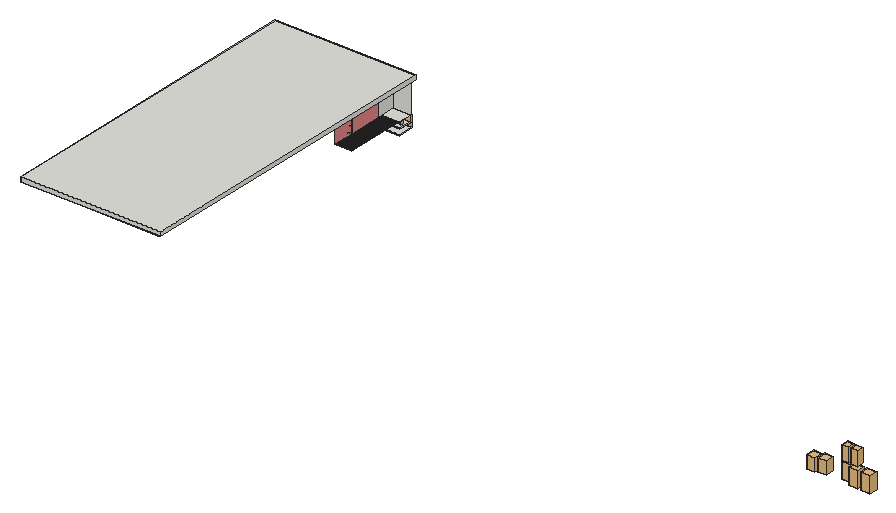
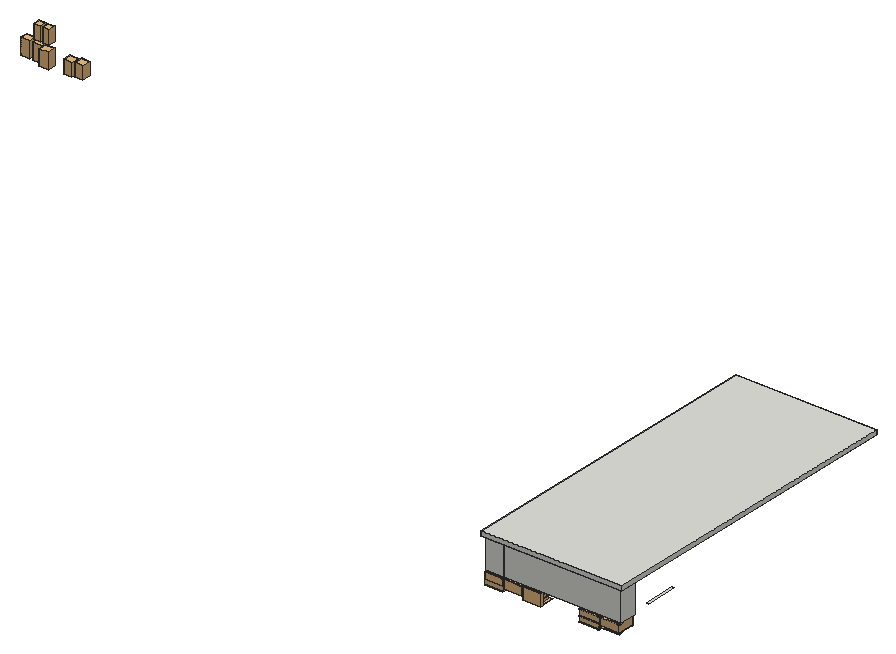
# SketchUp Ruby script. Lengths in inches.
U = 1.inch
M = Sketchup.active_model
def pt(a) = Geom::Point3d.new(a.map { |v| v * U })
def face(e, loops, mat)
  f = e.add_face(loops[0].map { |a| pt(a) })
  loops[1..].each { |l| e.add_face(l.map { |a| pt(a) }).erase! }
  f.material = f.back_material = mat if mat
  f
end
# faces: each face lists its corners as indices into pts; further lists are holes
def faces(e, pts, list, mat = nil) = list.each { |f| face(e, (f[0].is_a?(Array) ? f : [f]).map { |l| l.map { |i| pts[i] } }, mat) }
# xy, xz, yz: faces in a plane at the given z, y or x. An outline is a flat list of corners, or four numbers for a rectangle; further outlines are holes
def ring(l) = l.size == 4 ? [[l[0], l[1]], [l[2], l[1]], [l[2], l[3]], [l[0], l[3]]] : l.each_slice(2).to_a
def flat(e, list, mat, &to3) = list.each { |f| face(e, (f[0].is_a?(Array) ? f : [f]).map { |l| ring(l).map { |u, v| to3.(u, v) } }, mat) }
def xy(e, z, list, mat = nil) = flat(e, list, mat) { |x, y| [x, y, z] }
def xz(e, y, list, mat = nil) = flat(e, list, mat) { |x, z| [x, y, z] }
def yz(e, x, list, mat = nil) = flat(e, list, mat) { |y, z| [x, y, z] }
def lines(e, pts, list) = list.each { |a, b| e.add_line(pt(pts[a]), pt(pts[b])) }
# prism: a flat outline (further loops are holes) pulled along v
def prism(e, loops, v, mat = nil)
  f = face(e, loops, mat); d = Geom::Vector3d.new(v.map { |x| x * U })
  f.pushpull(f.normal.samedirection?(d) ? d.length : -d.length)
end
def box(e, o, s, mat = nil) = prism(e, [[o, [o[0] + s[0], o[1], o[2]], [o[0] + s[0], o[1] + s[1], o[2]], [o[0], o[1] + s[1], o[2]]]], [0, 0, s[2]], mat)
def at(x, y, z, deg = 0) = Geom::Transformation.translation(pt([x, y, z])) * Geom::Transformation.rotation(ORIGIN, Z_AXIS, deg.degrees)
def axes(o, x, y, z) = Geom::Transformation.new([*x, 0, *y, 0, *z, 0, *pt(o).to_a, 1])
def part(name) = M.definitions.add(name)
# library, detail: a bought-in or finely detailed component or shape, given as its bounding box
def library(name, o, s) = part(name).tap { |d| box(d.entities, o, s) }
def detail(e, o, s) = box(e.add_group.entities, o, s)
def put(e, d, t, mat = nil) = e.add_instance(d, t).tap { |i| i.material = mat if mat }
def group(e, t, mat = nil) = e.add_group.tap { |g| g.transformation = t; g.material = mat if mat }.entities
root = M.entities
M.materials.add("Generic\#1").color = [224, 133, 133]
M.materials.add("[0036_BurlyWood]").color = [222, 184, 135]
M.materials.add("[0134_DimGray]").color = [105, 105, 105]
M.materials.add("[0136_Charcoal]").color = [35, 35, 35]
M.materials.add("[Color M00]").color = [255, 255, 255]
c1 = library("Group\#42",[-0.5,-0.5,-0.1],[27.07,5.46,0.2])
c2 = library("Group\#45",[-0.5,-0.5,0],[25.0625,2.8125,15.73])
c3 = library("KITCHEN+ITEMS+(22)",[-8.24,-11.1,-0.01],[16.86,31.33,9.97])
c4 = library("Food+jars (2)",[-11.5,-3.52,0],[30.82,7.02,10])
c5 = library("Group\#41",[-0.5,-0.5,-0.1],[27.07,6.0625,0.2])
c6 = library("Group\#46",[-0.5,-0.5,0],[25.0625,7.1875,12.03])
c7 = library("KITCHEN+ITEMS+(3)",[-2.27,-9.02,0],[4.03,10.9,5.45])
c8 = library("Stocked cup rack",[0,0,0],[12.28,12.62,7.74])
c9 = library("Group\#47",[-0.5,-0.5,0],[25.0625,2.47,8.52])
c10 = library("Group\#43",[-0.5,-0.5,-0.1],[27.07,5.46,0.2])
c11 = library("Group\#8",[-92.73,64.66,378.72],[126.77,111.9,197.69])
c12 = library("Group\#3",[-457.8,68.7,378.69],[103.44,103.46,159.72])
c13 = library("Group\#12",[309.63,77.04,613.73],[136.79,86.78,171.39])
c14 = library("filizanka,+spodek+zestaw",[-38.08,-53.17,0],[37.3,56.83,6.3])
c15 = library("Food+jars (1)",[-3.15,-4.1,0],[15.4,16.05,11.47])
c16 = library("Group\#40",[-0.5,-0.5,-0.1],[27.07,5.5625,0.2])
c17 = library("Group\#44",[-0.5,-0.5,-0.1],[27.07,3.75,0.2])
c18 = part("Group\#105")
prism(c18.entities,[[[0.55,0,1.11],[0.51,0,1.03],[0.44,0,0.97],[0.36,0,0.9375],[0.28,0,0.92],[0.19,0,0.9375],[0.11,0,0.97],[0.05,0,1.03],[0,0,1.11],[0,0,0],[0.55,0,0]]],[0,0.79,0])
c19 = part("Cabinet bar pull")
put(c19.entities,c18,axes([0,1.42,1.36],[0,0,-1],[1,0,0],[0,-1,0]))
g1 = group(c19.entities,at(0,1.42,1.36))
prism(g1,[[[0,-1.28,-0.57],[0,-1.32,-0.53],[0,-1.35,-0.49],[0,-1.38,-0.4375],[0,-1.4,-0.39],[0,-1.41,-0.33],[0,-1.42,-0.28],[0,-1.41,-0.22],[0,-1.4,-0.17],[0,-1.38,-0.11],[0,-1.35,-0.0625],[0,-1.32,-0.02],[0,-1.28,0.02],[0,-1.19,0.02],[0,-1.11,0],[0,-1.03,-0.05],[0,-0.97,-0.11],[0,-0.9375,-0.19],[0,-0.92,-0.28],[0,-0.9375,-0.36],[0,-0.97,-0.44],[0,-1.03,-0.51],[0,-1.11,-0.55],[0,-1.19,-0.57]]],[13.07,0,0])
put(c19.entities,c18,axes([12.28,1.42,1.36],[0,0,-1],[1,0,0],[0,-1,0]))
c20 = library("10 (1)",[26.65,-5.45,122.92],[1.37,1.38,0.36])
c21 = library("Group\#4",[-210.76,89.58,378.69],[103.46,103.45,159.72])
c22 = library("Group\#2",[-332.7,68.71,378.69],[103.45,103.45,159.72])
c23 = library("Group\#9",[51.24,128.79,378.72],[113.79,95.47,197.69])
c24 = library("Group\#10",[179.9,72.7,378.72],[113.8,95.46,197.69])
c25 = library("Group\#11",[327.72,72.7,378.72],[113.79,95.46,197.69])
c26 = library("Group\#19",[85.42,84.74,613.85],[84,84,172.42])
c27 = library("Group\#20",[193.57,84.74,613.85],[84,84,172.39])
xy(root,63.79,[[166.14,409.25,190.2,429.57]],"[0036_BurlyWood]")
xy(root,64.03,[[36.39,410.57,62.46,425.11]])
xy(root,64.04,[[114.85,409.25,138.91,427.75]])
xy(root,64.85,[[166.14,409.25,190.2,429.57],[36.39,410.57,62.46,429.57]])
xy(root,64.85,[[114.85,409.25,138.91,429.57]],"[0036_BurlyWood]")
xy(root,67.74,[[140.5,407.75,164.56,423.38]],"[0036_BurlyWood]")
xy(root,67.8,[[8.77,407.75,34.84,424.5]],"[0036_BurlyWood]")
xy(root,68.58,[[140.5,407.75,164.56,429.57]])
xy(root,69.36,[[8.77,407.75,34.84,429.57]],"[0036_BurlyWood]")
xy(root,71.25,[[166.14,409.25,190.2,428.1]],"[0036_BurlyWood]")
xy(root,71.5,[[114.85,409.25,138.91,427.75],[36.39,410.57,62.46,425.11]])
xy(root,72.3125,[[166.14,409.25,190.2,429.57]])
xy(root,72.3125,[[114.85,409.25,138.91,429.57]],"[0036_BurlyWood]")
xy(root,72.32,[[36.39,410.57,62.46,429.57]])
xy(root,79.77,[[114.85,407.75,138.91,427.75],[140.5,407.75,164.56,423.38],[166.14,407.75,166.97,429.57],[166.97,407.75,190.2,428.1]],"[0036_BurlyWood]")
xy(root,79.79,[[8.77,407.75,34.84,425],[36.39,407.75,62.46,426.82]],"[0036_BurlyWood]")
xy(root,80.5625,[[7.99,407.75,166.97,427.75],[166.97,407.75,191,427.75]])
xy(root,80.5625,[[166.97,328.41,166.97,357.08,167.27,357.08,167.27,357.38,166.97,357.38,166.97,407.75,191,407.75,191,328.41],[7.99,403.75,7.99,407.75,166.97,407.75,166.97,403.75,135.48,403.75,135.48,404.05,135.18,404.05,135.18,403.75,103.68,403.75,103.68,404.05,103.38,404.05,103.38,403.75,71.88,403.75,71.88,404.05,71.58,404.05,71.58,403.75,40.09,403.75,40.09,404.05,39.79,404.05,39.79,403.75]],"[0136_Charcoal]")
xy(root,86.5625,[[4.74,342.29,7.99,384.54]])
xy(root,122.5625,[[4.74,0,4.74,431,194.24,431,194.24,0,191,0,191,427.75,7.99,427.75,7.99,0],[166.97,311,166.97,357.08,167.27,357.08,167.27,357.38,166.97,357.38,166.97,427.75,191,427.75,191,311],[7.99,403.75,7.99,427.75,166.97,427.75,166.97,403.75,135.48,403.75,135.48,404.05,135.18,404.05,135.18,403.75,103.68,403.75,103.68,404.05,103.38,404.05,103.38,403.75,71.88,403.75,71.88,404.05,71.58,404.05,71.58,403.75,40.09,403.75,40.09,404.05,39.79,404.05,39.79,403.75]])
xy(root,122.5625,[[[7.99,0,7.99,403.75,39.79,403.75,39.79,404.05,40.09,404.05,40.09,403.75,71.58,403.75,71.58,404.05,71.88,404.05,71.88,403.75,103.38,403.75,103.38,404.05,103.68,404.05,103.68,403.75,135.18,403.75,135.18,404.05,135.48,404.05,135.48,403.75,166.97,403.75,166.97,357.38,167.27,357.38,167.27,357.08,166.97,357.08,166.97,311,191,311,191,0],[33.53,377.24,34.16,377.32,34.75,377.57,35.25,377.95,35.64,378.46,35.88,379.05,35.97,379.68,35.88,380.31,35.64,380.9,35.25,381.4,34.75,381.79,34.16,382.03,33.53,382.11,32.9,382.03,32.31,381.79,31.81,381.4,31.42,380.9,31.17,380.31,31.09,379.68,31.17,379.05,31.42,378.46,31.81,377.95,32.31,377.57,32.9,377.32],[89.72,377.24,90.35,377.32,90.94,377.57,91.44,377.95,91.83,378.46,92.07,379.05,92.15,379.68,92.07,380.31,91.83,380.9,91.44,381.4,90.94,381.79,90.35,382.03,89.72,382.11,89.09,382.03,88.5,381.79,87.99,381.4,87.61,380.9,87.36,380.31,87.28,379.68,87.36,379.05,87.61,378.46,87.99,377.95,88.5,377.57,89.09,377.32],[141.03,377.24,141.66,377.32,142.25,377.57,142.75,377.95,143.14,378.46,143.38,379.05,143.47,379.68,143.38,380.31,143.14,380.9,142.75,381.4,142.25,381.79,141.66,382.03,141.03,382.11,140.4,382.03,139.81,381.79,139.31,381.4,138.92,380.9,138.67,380.31,138.59,379.68,138.67,379.05,138.92,378.46,139.31,377.95,139.81,377.57,140.4,377.32]]],"[Color M00]")
xy(root,123.25,[[33.53,377.24,32.9,377.32,32.31,377.57,31.81,377.95,31.42,378.46,31.17,379.05,31.09,379.68,31.17,380.31,31.42,380.9,31.81,381.4,32.31,381.79,32.9,382.03,33.53,382.11,34.16,382.03,34.75,381.79,35.25,381.4,35.64,380.9,35.88,380.31,35.97,379.68,35.88,379.05,35.64,378.46,35.25,377.95,34.75,377.57,34.16,377.32],[89.72,377.24,89.09,377.32,88.5,377.57,87.99,377.95,87.61,378.46,87.36,379.05,87.28,379.68,87.36,380.31,87.61,380.9,87.99,381.4,88.5,381.79,89.09,382.03,89.72,382.11,90.35,382.03,90.94,381.79,91.44,381.4,91.83,380.9,92.07,380.31,92.15,379.68,92.07,379.05,91.83,378.46,91.44,377.95,90.94,377.57,90.35,377.32],[141.03,377.24,140.4,377.32,139.81,377.57,139.31,377.95,138.92,378.46,138.67,379.05,138.59,379.68,138.67,380.31,138.92,380.9,139.31,381.4,139.81,381.79,140.4,382.03,141.03,382.11,141.66,382.03,142.25,381.79,142.75,381.4,143.14,380.9,143.38,380.31,143.47,379.68,143.38,379.05,143.14,378.46,142.75,377.95,142.25,377.57,141.66,377.32]])
xy(root,128.5625,[[4.74,0,194.24,431]])
xz(root,0,[[4.74,122.5625,194.24,128.5625]])
xz(root,357.08,[[166.97,80.5625,167.27,122.5625]])
xz(root,357.38,[[166.97,80.5625,167.27,122.5625]])
xz(root,403.75,[[7.99,80.5625,39.79,122.5625],[40.09,80.5625,71.58,122.5625],[71.88,80.5625,103.38,122.5625],[103.68,80.5625,135.18,122.5625],[135.48,80.5625,166.97,122.5625]],"Generic\#1")
xz(root,404.05,[[39.79,80.5625,40.09,122.5625],[71.58,80.5625,71.88,122.5625],[103.38,80.5625,103.68,122.5625],[135.18,80.5625,135.48,122.5625]])
xz(root,407.75,[[[7.99,68.58,35.61,80.5625],[8.77,69.36,34.84,79.79]]])
xz(root,407.75,[[140.5,67.74,164.56,68.58]],"[0134_DimGray]")
xz(root,409.25,[[166.14,63.79,190.2,64.85],[114.85,64.04,138.91,64.85],[166.14,71.25,190.2,72.3125],[114.85,71.5,138.91,72.3125]],"[0134_DimGray]")
xz(root,410.57,[[36.39,64.03,62.46,64.85],[36.39,71.5,62.46,72.32]],"[0134_DimGray]")
xz(root,427.75,[[7.99,80.5625,166.97,122.5625],[166.97,80.5625,191,122.5625]])
xz(root,429.57,[[166.14,63.79,190.2,64.85],[114.85,64.04,138.91,64.85],[166.14,71.25,190.2,72.3125],[114.85,71.5,138.91,72.3125]])
xz(root,429.57,[[36.39,64.85,62.46,71.5],[114.85,64.85,138.91,71.5],[166.14,64.85,190.2,71.25],[140.5,68.58,164.56,79.77],[8.77,69.36,34.84,79.79],
  [114.85,72.3125,138.91,79.77],[166.14,72.3125,190.2,79.77],[36.39,72.32,62.46,79.79]],"[0036_BurlyWood]")
xz(root,431,[[4.74,122.5625,194.24,128.5625]])
yz(root,4.74,[[0,122.5625,431,128.5625]])
yz(root,7.99,[[403.75,80.5625,427.75,122.5625]])
yz(root,8.77,[[407.75,69.36,429.57,79.79]],"[0036_BurlyWood]")
yz(root,34.84,[[407.75,69.36,429.57,79.79]],"[0036_BurlyWood]")
yz(root,39.79,[[403.75,80.5625,404.05,122.5625]])
yz(root,40.09,[[403.75,80.5625,404.05,122.5625]])
yz(root,71.58,[[403.75,80.5625,404.05,122.5625]])
yz(root,71.88,[[403.75,80.5625,404.05,122.5625]])
yz(root,103.38,[[403.75,80.5625,404.05,122.5625]])
yz(root,103.68,[[403.75,80.5625,404.05,122.5625]])
yz(root,114.85,[[409.25,64.04,429.57,64.85],[409.25,71.5,429.57,72.3125]])
yz(root,135.18,[[403.75,80.5625,404.05,122.5625]])
yz(root,135.48,[[403.75,80.5625,404.05,122.5625]])
yz(root,138.91,[[409.25,64.04,429.57,64.85],[409.25,71.5,429.57,72.3125]])
yz(root,140.5,[[407.75,68.58,429.57,79.77]],"[0036_BurlyWood]")
yz(root,164.56,[[407.75,68.58,429.57,79.77]],"[0036_BurlyWood]")
yz(root,166.14,[[409.25,63.79,429.57,64.85],[409.25,71.25,429.57,72.3125]])
yz(root,166.97,[[403.75,80.5625,427.75,122.5625]])
yz(root,166.97,[[328.41,80.5625,357.08,122.5625],[357.38,80.5625,403.75,122.5625]],"Generic\#1")
yz(root,167.27,[[357.08,80.5625,357.38,122.5625]])
yz(root,190.2,[[409.25,63.79,429.57,64.85],[409.25,71.25,429.57,72.3125]])
yz(root,194.24,[[0,122.5625,431,128.5625]])
p = [[33.53,377.24,122.5625],[32.9,377.32,122.5625],[32.9,377.32,123.25],[33.53,377.24,123.25],[34.16,377.32,122.5625],[34.16,377.32,123.25],
  [89.72,377.24,122.5625],[89.09,377.32,122.5625],[89.09,377.32,123.25],[89.72,377.24,123.25],[90.35,377.32,122.5625],[90.35,377.32,123.25],
  [141.03,377.24,122.5625],[140.4,377.32,122.5625],[140.4,377.32,123.25],[141.03,377.24,123.25],[141.66,377.32,122.5625],[141.66,377.32,123.25],
  [32.31,377.57,122.5625],[32.31,377.57,123.25],[34.75,377.57,122.5625],[34.75,377.57,123.25],[88.5,377.57,122.5625],[88.5,377.57,123.25],
  [90.94,377.57,122.5625],[90.94,377.57,123.25],[139.81,377.57,122.5625],[139.81,377.57,123.25],[142.25,377.57,122.5625],[142.25,377.57,123.25],
  [31.81,377.95,122.5625],[31.81,377.95,123.25],[35.25,377.95,122.5625],[35.25,377.95,123.25],[87.99,377.95,122.5625],[87.99,377.95,123.25],
  [91.44,377.95,122.5625],[91.44,377.95,123.25],[139.31,377.95,122.5625],[139.31,377.95,123.25],[142.75,377.95,122.5625],[142.75,377.95,123.25],
  [31.42,378.46,122.5625],[31.42,378.46,123.25],[35.64,378.46,122.5625],[35.64,378.46,123.25],[87.61,378.46,122.5625],[87.61,378.46,123.25],
  [91.83,378.46,122.5625],[91.83,378.46,123.25],[138.92,378.46,122.5625],[138.92,378.46,123.25],[143.14,378.46,122.5625],[143.14,378.46,123.25],
  [31.17,379.05,122.5625],[31.17,379.05,123.25],[35.88,379.05,122.5625],[35.88,379.05,123.25],[87.36,379.05,122.5625],[87.36,379.05,123.25],
  [92.07,379.05,122.5625],[92.07,379.05,123.25],[138.67,379.05,122.5625],[138.67,379.05,123.25],[143.38,379.05,122.5625],[143.38,379.05,123.25],
  [31.09,379.68,122.5625],[31.09,379.68,123.25],[35.97,379.68,122.5625],[35.97,379.68,123.25],[87.28,379.68,122.5625],[87.28,379.68,123.25],
  [92.15,379.68,122.5625],[92.15,379.68,123.25],[138.59,379.68,122.5625],[138.59,379.68,123.25],[143.47,379.68,122.5625],[143.47,379.68,123.25],
  [31.17,380.31,122.5625],[31.17,380.31,123.25],[35.88,380.31,122.5625],[35.88,380.31,123.25],[87.36,380.31,122.5625],[87.36,380.31,123.25],
  [92.07,380.31,122.5625],[92.07,380.31,123.25],[138.67,380.31,122.5625],[138.67,380.31,123.25],[143.38,380.31,122.5625],[143.38,380.31,123.25],
  [31.42,380.9,122.5625],[31.42,380.9,123.25],[35.64,380.9,122.5625],[35.64,380.9,123.25],[87.61,380.9,122.5625],[87.61,380.9,123.25],
  [91.83,380.9,122.5625],[91.83,380.9,123.25],[138.92,380.9,122.5625],[138.92,380.9,123.25],[143.14,380.9,122.5625],[143.14,380.9,123.25],
  [31.81,381.4,122.5625],[31.81,381.4,123.25],[35.25,381.4,122.5625],[35.25,381.4,123.25],[87.99,381.4,122.5625],[87.99,381.4,123.25],
  [91.44,381.4,122.5625],[91.44,381.4,123.25],[139.31,381.4,122.5625],[139.31,381.4,123.25],[142.75,381.4,122.5625],[142.75,381.4,123.25],
  [32.31,381.79,122.5625],[32.31,381.79,123.25],[34.75,381.79,122.5625],[34.75,381.79,123.25],[88.5,381.79,122.5625],[88.5,381.79,123.25],
  [90.94,381.79,122.5625],[90.94,381.79,123.25],[139.81,381.79,122.5625],[139.81,381.79,123.25],[142.25,381.79,122.5625],[142.25,381.79,123.25],
  [32.9,382.03,122.5625],[32.9,382.03,123.25],[34.16,382.03,122.5625],[34.16,382.03,123.25],[89.09,382.03,122.5625],[89.09,382.03,123.25],
  [90.35,382.03,122.5625],[90.35,382.03,123.25],[140.4,382.03,122.5625],[140.4,382.03,123.25],[141.66,382.03,122.5625],[141.66,382.03,123.25],
  [33.53,382.11,122.5625],[33.53,382.11,123.25],[89.72,382.11,122.5625],[89.72,382.11,123.25],[141.03,382.11,122.5625],[141.03,382.11,123.25],
  [191,328.41,80.5625],[194.22,328.41,80.5625]]
faces(root,p,[[0,1,2,3],[4,0,3,5],[6,7,8,9],[10,6,9,11],[12,13,14,15],[16,12,15,17],[1,18,19,2],[20,4,5,21],
  [7,22,23,8],[24,10,11,25],[13,26,27,14],[28,16,17,29],[18,30,31,19],[32,20,21,33],[22,34,35,23],[36,24,25,37],
  [26,38,39,27],[40,28,29,41],[30,42,43,31],[44,32,33,45],[34,46,47,35],[48,36,37,49],[38,50,51,39],[52,40,41,53],
  [42,54,55,43],[56,44,45,57],[46,58,59,47],[60,48,49,61],[50,62,63,51],[64,52,53,65],[54,66,67,55],[68,56,57,69],
  [58,70,71,59],[72,60,61,73],[62,74,75,63],[76,64,65,77],[66,78,79,67],[80,68,69,81],[70,82,83,71],[84,72,73,85],
  [74,86,87,75],[88,76,77,89],[78,90,91,79],[92,80,81,93],[82,94,95,83],[96,84,85,97],[86,98,99,87],[100,88,89,101],
  [90,102,103,91],[104,92,93,105],[94,106,107,95],[108,96,97,109],[98,110,111,99],[112,100,101,113],[102,114,115,103],[116,104,105,117],
  [106,118,119,107],[120,108,109,121],[110,122,123,111],[124,112,113,125],[114,126,127,115],[128,116,117,129],[118,130,131,119],[132,120,121,133],
  [122,134,135,123],[136,124,125,137],[126,138,139,127],[138,128,129,139],[130,140,141,131],[140,132,133,141],[134,142,143,135],[142,136,137,143]])
lines(root,p,[[144,145]])
put(root,c1,at(36.39,425.11,64.03))
put(root,c2,at(114.85,427.75,64.04))
put(root,c3,axes([123.63,418.28,64.85],[0,-0.5,0],[0.5,0,0],[0,0,0.5]))
put(root,c4,axes([46.03,416.08,64.85],[0.6216,0,0],[0,0.6216,0],[0,0,0.6216]))
put(root,c5,at(8.77,424.5,67.8))
put(root,c6,at(140.5,423.38,67.74))
put(root,c7,at(149.06,415.51,68.58,90))
put(root,c8,at(16.67,407.75,69.36))
put(root,c9,at(166.14,428.1,71.25))
put(root,c10,at(36.39,425.11,71.5))
put(root,c11,axes([173.12,414.43,60.1],[0.0319,0,0],[0,0.0319,0],[0,0,0.0319]))
put(root,c12,axes([194.85,413.9,56.4375],[0.0418,0,0],[0,0.0418,0],[0,0,0.0418]))
put(root,c13,axes([172.16,414.4,52.7],[0.0319,0,0],[0,0.0319,0],[0,0,0.0319]))
put(root,c14,axes([137.36,408.93,72.3125],[0,-0.42,0],[0.42335,0,0],[0,0,0.56]))
put(root,c15,axes([55.98,420.42,72.32],[-0.46,0,0],[0,-0.46,0],[0,0,0.46]))
put(root,c15,axes([48.71,419.73,72.32],[-0.46,0,0],[0,-0.46,0],[0,0,0.46]))
put(root,c16,at(8.77,425,79.79))
put(root,c17,at(36.39,426.82,79.79))
put(root,c19,axes([135.88,402.11,90.27],[0,0,-0.6547],[0,1.16,0],[1.16,0,0]))
put(root,c19,axes([132.69,402.11,90.27],[0,0,-0.6547],[0,1.16,0],[1.16,0,0]))
put(root,c19,axes([35.63,402.11,90.27],[0,0,-0.6547],[0,1.16,0],[1.16,0,0]))
put(root,c19,axes([68.88,402.11,90.27],[0,0,-0.6547],[0,1.16,0],[1.16,0,0]))
put(root,c19,axes([72.32,402.11,90.27],[0,0,-0.6547],[0,1.16,0],[1.16,0,0]))
put(root,c19,axes([165.33,354.66,91.84],[0,0,-0.6547],[1.16,0,0],[0,-1.16,0]))
put(root,c19,axes([165.33,360.84,91.84],[0,0,-0.6547],[1.16,0,0],[0,-1.16,0]))
put(root,c20,axes([-76.16,398.39,-371.7],[4.01489,0,0],[0,4.01489,0],[0,0,4.01489]))
put(root,c20,axes([-19.59,398.39,-371.7],[4.01489,0,0],[0,4.01489,0],[0,0,4.01489]))
put(root,c20,axes([30.97,398.39,-371.7],[4.01489,0,0],[0,4.01489,0],[0,0,4.01489]))
put(root,c21,axes([1124.79,-32.09,123.83],[0.11,0,0],[0,0.11,0],[0,0,0.11]))
put(root,c22,axes([1124.79,-32.09,123.83],[0.11,0,0],[0,0.11,0],[0,0,0.11]))
put(root,c23,axes([1124.79,-32.09,123.83],[0.11,0,0],[0,0.11,0],[0,0,0.11]))
put(root,c24,axes([1124.79,-32.09,123.83],[0.11,0,0],[0,0.11,0],[0,0,0.11]))
put(root,c25,axes([1124.79,-32.09,123.83],[0.11,0,0],[0,0.11,0],[0,0,0.11]))
put(root,c26,axes([1124.79,-32.09,123.83],[0.11,0,0],[0,0.11,0],[0,0,0.11]))
put(root,c27,axes([1124.79,-32.09,123.83],[0.11,0,0],[0,0.11,0],[0,0,0.11]))
